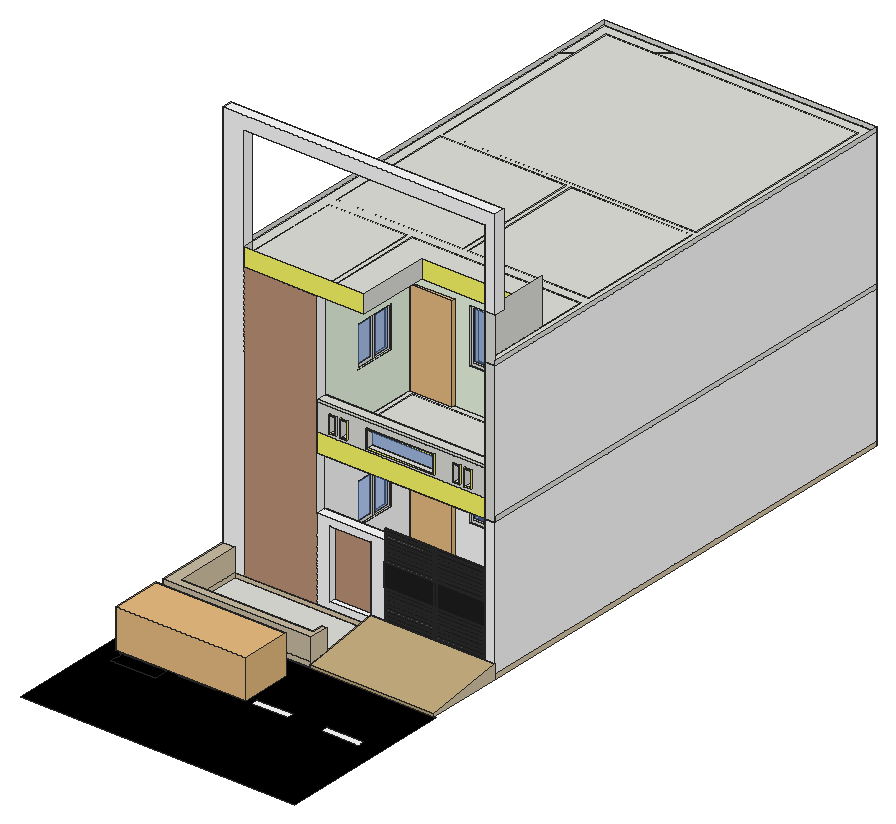
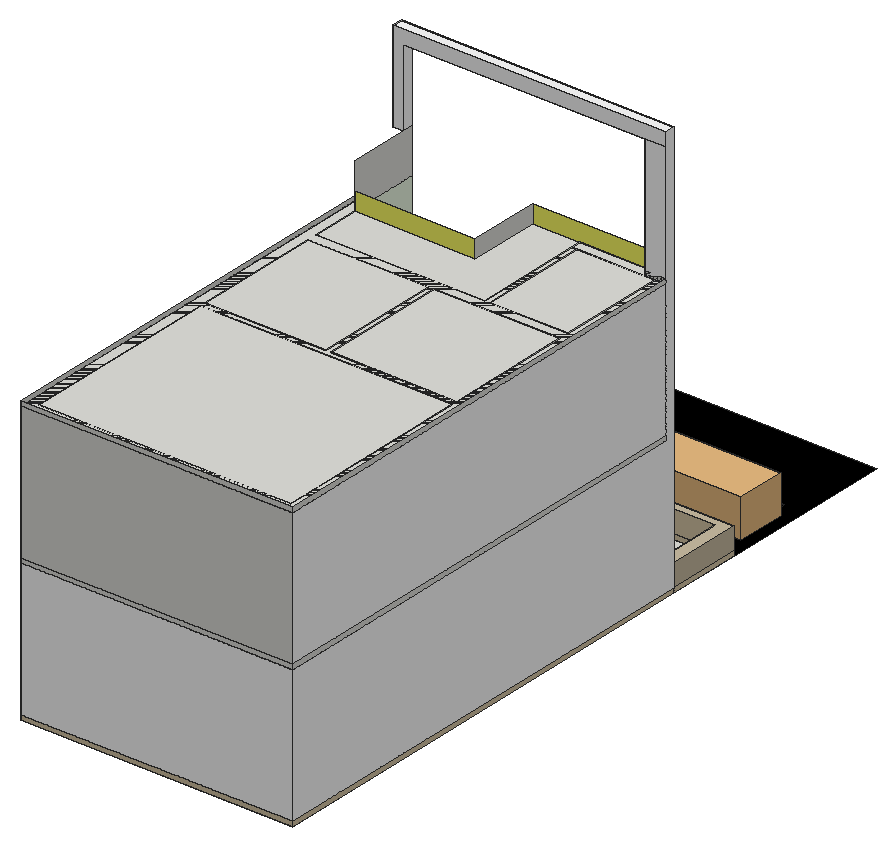
# SketchUp Ruby script. Lengths in inches.
U = 1.inch
M = Sketchup.active_model
def pt(a) = Geom::Point3d.new(a.map { |v| v * U })
def face(e, loops, mat)
  f = e.add_face(loops[0].map { |a| pt(a) })
  loops[1..].each { |l| e.add_face(l.map { |a| pt(a) }).erase! }
  f.material = f.back_material = mat if mat
  f
end
# faces: each face lists its corners as indices into pts; further lists are holes
def faces(e, pts, list, mat = nil) = list.each { |f| face(e, (f[0].is_a?(Array) ? f : [f]).map { |l| l.map { |i| pts[i] } }, mat) }
# xy, xz, yz: faces in a plane at the given z, y or x. An outline is a flat list of corners, or four numbers for a rectangle; further outlines are holes
def ring(l) = l.size == 4 ? [[l[0], l[1]], [l[2], l[1]], [l[2], l[3]], [l[0], l[3]]] : l.each_slice(2).to_a
def flat(e, list, mat, &to3) = list.each { |f| face(e, (f[0].is_a?(Array) ? f : [f]).map { |l| ring(l).map { |u, v| to3.(u, v) } }, mat) }
def xy(e, z, list, mat = nil) = flat(e, list, mat) { |x, y| [x, y, z] }
def xz(e, y, list, mat = nil) = flat(e, list, mat) { |x, z| [x, y, z] }
def yz(e, x, list, mat = nil) = flat(e, list, mat) { |y, z| [x, y, z] }
def lines(e, pts, list) = list.each { |a, b| e.add_line(pt(pts[a]), pt(pts[b])) }
# prism: a flat outline (further loops are holes) pulled along v
def prism(e, loops, v, mat = nil)
  f = face(e, loops, mat); d = Geom::Vector3d.new(v.map { |x| x * U })
  f.pushpull(f.normal.samedirection?(d) ? d.length : -d.length)
end
def box(e, o, s, mat = nil) = prism(e, [[o, [o[0] + s[0], o[1], o[2]], [o[0] + s[0], o[1] + s[1], o[2]], [o[0], o[1] + s[1], o[2]]]], [0, 0, s[2]], mat)
def at(x, y, z, deg = 0) = Geom::Transformation.translation(pt([x, y, z])) * Geom::Transformation.rotation(ORIGIN, Z_AXIS, deg.degrees)
def axes(o, x, y, z) = Geom::Transformation.new([*x, 0, *y, 0, *z, 0, *pt(o).to_a, 1])
def part(name) = M.definitions.add(name)
# library, detail: a bought-in or finely detailed component or shape, given as its bounding box
def library(name, o, s) = part(name).tap { |d| box(d.entities, o, s) }
def detail(e, o, s) = box(e.add_group.entities, o, s)
def put(e, d, t, mat = nil) = e.add_instance(d, t).tap { |i| i.material = mat if mat }
def group(e, t, mat = nil) = e.add_group.tap { |g| g.transformation = t; g.material = mat if mat }.entities
root = M.entities
M.materials.add("Color_008").color = [30, 30, 30]
M.materials.add("[0055_LightGoldenrodYellow]").color = [250, 250, 210]
M.materials.add("[0131_Silver]").color = [192, 192, 192]
M.materials.add("[0134_DimGray]").color = [105, 105, 105]
M.materials.add("[Color A01]").color = [191, 147, 119]
M.materials.add("[Color C01]").color = [191, 147, 119]
M.materials.add("[Color E03]").color = [255, 255, 104]
M.materials.add("[Color M00]").color = [255, 255, 255]
M.materials.add("[Color M09]").color = [0, 0, 0]
M.materials.add("[Concrete Tile]").color = [203, 190, 164]
M.materials.add("[Field Square Tile]").color = [217, 201, 169]
M.materials.add("[Roofing Slate Tan]").color = [200, 175, 128]
M.materials.add("[Tile Limestone Large]").color = [238, 251, 230]
M.materials.add("[Translucent Glass Blue]").color = [100, 149, 237]
M.materials["[Translucent Glass Blue]"].alpha = 0.5
c1 = library("Passenger car",[0,0,0],[114.57,43.85,34.01])
c2 = library("Untitled",[-28.23,109.14,0],[52,7.35,84])
c3 = part("Gate slat")
box(c3.entities,[0,0,-2.03],[1.97,0.97,40.94])
c4 = part("Gate frame member")
box(c4.entities,[0,0,0],[1.9,0.97,93.54])
c5 = part("Gate slat \#1")
box(c5.entities,[2.95,0,-2.03],[0.99,0.97,40.94])
c6 = part("Slatted gate")
p = [[42.85,0.97,43.31],[42.85,0.97,44.29]]
lines(c6.entities,p,[[0,1]])
put(c6.entities,c3,axes([3.9375,0,86.61],[0,0,-1],[0,1,0],[1,0,0]),"Color_008")
put(c6.entities,c4,axes([87.6,0,0],[1,0,0],[0,1,0],[0,0,0.92593]),"Color_008")
put(c6.entities,c3,axes([48.6875,0,86.61],[0,0,-1],[0,1,0],[1,0,0]),"Color_008")
put(c6.entities,c4,axes([0,0,0],[1,0,0],[0,1,0],[0,0,0.92593]),"Color_008")
put(c6.entities,c4,axes([42.85,0,0],[1,0,0],[0,1,0],[0,0,0.92593]),"Color_008")
put(c6.entities,c4,axes([44.75,0,0],[1,0,0],[0,1,0],[0,0,0.92593]),"Color_008")
put(c6.entities,c5,axes([3.9375,0,87.11],[0,0,-1],[0,1,0],[1,0,0]),"[0134_DimGray]")
put(c6.entities,c5,axes([48.6875,0,87.11],[0,0,-1],[0,1,0],[1,0,0]),"[0134_DimGray]")
put(c6.entities,c3,axes([48.6875,0,82.68],[0,0,-1],[0,1,0],[1,0,0]),"Color_008")
put(c6.entities,c5,axes([48.6875,0,83.17],[0,0,-1],[0,1,0],[1,0,0]),"[0134_DimGray]")
put(c6.entities,c5,axes([3.9375,0,83.17],[0,0,-1],[0,1,0],[1,0,0]),"[0134_DimGray]")
put(c6.entities,c3,axes([3.9375,0,82.68],[0,0,-1],[0,1,0],[1,0,0]),"Color_008")
put(c6.entities,c5,axes([48.6875,0,75.3],[0,0,-1],[0,1,0],[1,0,0]),"[0134_DimGray]")
put(c6.entities,c3,axes([48.6875,0,78.74],[0,0,-1],[0,1,0],[1,0,0]),"Color_008")
put(c6.entities,c3,axes([48.6875,0,74.8],[0,0,-1],[0,1,0],[1,0,0]),"Color_008")
put(c6.entities,c5,axes([48.6875,0,79.23],[0,0,-1],[0,1,0],[1,0,0]),"[0134_DimGray]")
put(c6.entities,c5,axes([3.9375,0,75.3],[0,0,-1],[0,1,0],[1,0,0]),"[0134_DimGray]")
put(c6.entities,c3,axes([3.9375,0,78.74],[0,0,-1],[0,1,0],[1,0,0]),"Color_008")
put(c6.entities,c5,axes([3.9375,0,79.23],[0,0,-1],[0,1,0],[1,0,0]),"[0134_DimGray]")
put(c6.entities,c3,axes([3.9375,0,74.8],[0,0,-1],[0,1,0],[1,0,0]),"Color_008")
put(c6.entities,c5,axes([48.6875,0,67.42],[0,0,-1],[0,1,0],[1,0,0]),"[0134_DimGray]")
put(c6.entities,c5,axes([3.9375,0,63.48],[0,0,-1],[0,1,0],[1,0,0]),"[0134_DimGray]")
put(c6.entities,c5,axes([48.6875,0,71.36],[0,0,-1],[0,1,0],[1,0,0]),"[0134_DimGray]")
put(c6.entities,c5,axes([3.9375,0,67.42],[0,0,-1],[0,1,0],[1,0,0]),"[0134_DimGray]")
put(c6.entities,c3,axes([3.9375,0,70.87],[0,0,-1],[0,1,0],[1,0,0]),"Color_008")
put(c6.entities,c3,axes([48.6875,0,70.87],[0,0,-1],[0,1,0],[1,0,0]),"Color_008")
put(c6.entities,c3,axes([48.6875,0,66.93],[0,0,-1],[0,1,0],[1,0,0]),"Color_008")
put(c6.entities,c3,axes([48.6875,0,59.06],[0,0,-1],[0,1,0],[1,0,0]),"Color_008")
put(c6.entities,c3,axes([3.9375,0,55.12],[0,0,-1],[0,1,0],[1,0,0]),"Color_008")
put(c6.entities,c3,axes([3.9375,0,62.99],[0,0,-1],[0,1,0],[1,0,0]),"Color_008")
put(c6.entities,c5,axes([3.9375,0,59.55],[0,0,-1],[0,1,0],[1,0,0]),"[0134_DimGray]")
put(c6.entities,c3,axes([3.9375,0,66.93],[0,0,-1],[0,1,0],[1,0,0]),"Color_008")
put(c6.entities,c3,axes([48.6875,0,62.99],[0,0,-1],[0,1,0],[1,0,0]),"Color_008")
put(c6.entities,c5,axes([48.6875,0,59.55],[0,0,-1],[0,1,0],[1,0,0]),"[0134_DimGray]")
put(c6.entities,c5,axes([48.6875,0,63.48],[0,0,-1],[0,1,0],[1,0,0]),"[0134_DimGray]")
put(c6.entities,c3,axes([3.9375,0,59.06],[0,0,-1],[0,1,0],[1,0,0]),"Color_008")
put(c6.entities,c5,axes([3.9375,0,71.36],[0,0,-1],[0,1,0],[1,0,0]),"[0134_DimGray]")
put(c6.entities,c5,axes([3.9375,0,33.96],[0,0,-1],[0,1,0],[1,0,0]),"[0134_DimGray]")
put(c6.entities,c5,axes([48.6875,0,33.96],[0,0,-1],[0,1,0],[1,0,0]),"[0134_DimGray]")
put(c6.entities,c3,axes([3.9375,0,29.53],[0,0,-1],[0,1,0],[1,0,0]),"Color_008")
put(c6.entities,c5,axes([3.9375,0,26.08],[0,0,-1],[0,1,0],[1,0,0]),"[0134_DimGray]")
put(c6.entities,c3,axes([3.9375,0,33.46],[0,0,-1],[0,1,0],[1,0,0]),"Color_008")
put(c6.entities,c3,axes([48.6875,0,29.53],[0,0,-1],[0,1,0],[1,0,0]),"Color_008")
put(c6.entities,c5,axes([48.6875,0,30.02],[0,0,-1],[0,1,0],[1,0,0]),"[0134_DimGray]")
put(c6.entities,c3,axes([3.9375,0,25.59],[0,0,-1],[0,1,0],[1,0,0]),"Color_008")
put(c6.entities,c3,axes([48.6875,0,25.59],[0,0,-1],[0,1,0],[1,0,0]),"Color_008")
put(c6.entities,c3,axes([48.6875,0,33.46],[0,0,-1],[0,1,0],[1,0,0]),"Color_008")
put(c6.entities,c3,axes([3.9375,0,49.7],[0,0,-1],[0,1,0],[1,0,0]),"Color_008")
put(c6.entities,c5,axes([48.6875,0,26.08],[0,0,-1],[0,1,0],[1,0,0]),"[0134_DimGray]")
put(c6.entities,c5,axes([3.9375,0,30.02],[0,0,-1],[0,1,0],[1,0,0]),"[0134_DimGray]")
put(c6.entities,c3,axes([3.9375,0,5.91],[0,0,-1],[0,1,0],[1,0,0]),"Color_008")
put(c6.entities,c3,axes([48.6875,0,13.78],[0,0,-1],[0,1,0],[1,0,0]),"Color_008")
put(c6.entities,c5,axes([48.6875,0,10.33],[0,0,-1],[0,1,0],[1,0,0]),"[0134_DimGray]")
put(c6.entities,c5,axes([3.9375,0,6.4],[0,0,-1],[0,1,0],[1,0,0]),"[0134_DimGray]")
put(c6.entities,c3,axes([3.9375,0,13.78],[0,0,-1],[0,1,0],[1,0,0]),"Color_008")
put(c6.entities,c3,axes([48.6875,0,21.65],[0,0,-1],[0,1,0],[1,0,0]),"Color_008")
put(c6.entities,c3,axes([48.6875,0,5.91],[0,0,-1],[0,1,0],[1,0,0]),"Color_008")
put(c6.entities,c5,axes([48.6875,0,22.15],[0,0,-1],[0,1,0],[1,0,0]),"[0134_DimGray]")
put(c6.entities,c3,axes([48.6875,0,1.97],[0,0,-1],[0,1,0],[1,0,0]),"Color_008")
put(c6.entities,c3,axes([48.6875,0,9.84],[0,0,-1],[0,1,0],[1,0,0]),"Color_008")
put(c6.entities,c5,axes([48.6875,0,6.4],[0,0,-1],[0,1,0],[1,0,0]),"[0134_DimGray]")
put(c6.entities,c3,axes([3.9375,0,9.84],[0,0,-1],[0,1,0],[1,0,0]),"Color_008")
put(c6.entities,c5,axes([3.9375,0,10.33],[0,0,-1],[0,1,0],[1,0,0]),"[0134_DimGray]")
put(c6.entities,c5,axes([3.9375,0,22.15],[0,0,-1],[0,1,0],[1,0,0]),"[0134_DimGray]")
put(c6.entities,c3,axes([3.9375,0,1.97],[0,0,-1],[0,1,0],[1,0,0]),"Color_008")
put(c6.entities,c5,axes([3.9375,0,18.21],[0,0,-1],[0,1,0],[1,0,0]),"[0134_DimGray]")
put(c6.entities,c5,axes([3.9375,0,14.27],[0,0,-1],[0,1,0],[1,0,0]),"[0134_DimGray]")
put(c6.entities,c3,axes([3.9375,0,21.65],[0,0,-1],[0,1,0],[1,0,0]),"Color_008")
put(c6.entities,c5,axes([48.6875,0,18.21],[0,0,-1],[0,1,0],[1,0,0]),"[0134_DimGray]")
put(c6.entities,c3,axes([3.9375,0,17.72],[0,0,-1],[0,1,0],[1,0,0]),"Color_008")
put(c6.entities,c3,axes([48.6875,0,17.72],[0,0,-1],[0,1,0],[1,0,0]),"Color_008")
put(c6.entities,c5,axes([48.6875,0,14.27],[0,0,-1],[0,1,0],[1,0,0]),"[0134_DimGray]")
put(c6.entities,c3,axes([3.9375,0,44.29],[0,0,-1],[0,1,0],[1,0,0]),"Color_008")
put(c6.entities,c3,axes([3.9375,0,38.88],[0,0,-1],[0,1,0],[1,0,0]),"Color_008")
put(c6.entities,c3,axes([48.6875,0,49.7],[0,0,-1],[0,1,0],[1,0,0]),"Color_008")
put(c6.entities,c3,axes([48.6875,0,44.29],[0,0,-1],[0,1,0],[1,0,0]),"Color_008")
put(c6.entities,c3,axes([48.6875,0,38.88],[0,0,-1],[0,1,0],[1,0,0]),"Color_008")
put(c6.entities,c3,axes([48.6875,0,55.12],[0,0,-1],[0,1,0],[1,0,0]),"Color_008")
c7 = part("Glass panel \#1")
box(c7.entities,[0,0,-1.97],[52.81,0.39,23.62])
c8 = part("Glass panel")
box(c8.entities,[0,0,-9.84],[39.64,0.39,36.58])
c9 = part("Janela aluminio")
xy(c9.entities,0,[[0,0,47.24,1.57],[23.62,1.57,47.24,2.76],[0,2.76,25.98,3.9375],[0,3.9375,47.24,5.91]])
xy(c9.entities,43.31,[[0,0,47.24,1.57],[23.62,1.57,47.24,2.76],[0,2.76,0,5.91,47.24,5.91,47.24,3.9375,25.98,3.9375,25.98,2.76],[25.98,2.76,47.24,3.9375]])
xz(c9.entities,1.57,[[0,0,23.62,0,23.62,41.34,21.26,41.34,21.26,1.97,1.97,1.97,1.97,41.34,23.62,41.34,23.62,43.31,0,43.31],[[23.62,0,47.24,43.31],[25.7,1.97,45.28,41.34]]])
xz(c9.entities,2.76,[[[0,0,23.62,43.31],[2.36,2.36,21.26,40.94]],[23.62,0,25.98,43.31]])
xz(c9.entities,2.76,[[2.36,2.36,21.26,40.94]],"[Translucent Glass Blue]")
xz(c9.entities,3.9375,[[25.98,0,25.98,2.36,44.88,2.36,44.88,40.94,25.98,40.94,25.98,43.31,47.24,43.31,47.24,0]])
xz(c9.entities,3.9375,[[25.98,2.36,44.88,40.94]],"[Translucent Glass Blue]")
yz(c9.entities,0,[[0,0,1.57,43.31],[2.76,0,5.91,43.31]])
yz(c9.entities,23.62,[[1.57,0,2.76,43.31]])
yz(c9.entities,25.98,[[2.76,0,3.9375,43.31]])
yz(c9.entities,47.24,[[0,0,1.57,43.31],[1.57,0,2.76,43.31],[3.9375,0,5.91,43.31]])
xy(root,19.1,[[0,156,130.5,223.5]])
xy(root,19.1,[[66.31,91.44,99.35,98.41],[14.46,91.5,47.5,98.47],[129.67,91.8125,162.71,98.78],[191.22,91.96,224.26,98.93]],"[Color M00]")
xy(root,19.1,[[[0,0,242,156],[16.76,78.5,16.76,91.5,14.46,91.5,14.46,98.47,47.5,98.47,47.5,91.5,56.26,91.5,56.26,78.5],[66.31,91.44,99.35,98.41],[129.67,91.8125,162.71,98.78],[191.22,91.96,224.26,98.93]],[16.76,78.5,56.26,91.5]],"[Color M09]")
xy(root,267.1,[[18,223.5,18,232.5,0,232.5,0,643.5,240,643.5,240,223.5,231,223.5,231,286.5,124.5,286.5,124.5,223.5]])
xz(root,223.5,[[231,267.1,240,307.1]])
xz(root,223.5,[[18,267.1,124.5,283.1]],"[Color E03]")
xz(root,232.5,[[0,267.1,18,271.1]])
xz(root,286.5,[[124.5,267.1,231,283.1]],"[Color E03]")
xz(root,643.5,[[0,267.1,240,271.1]])
yz(root,0,[[232.5,267.1,643.5,271.1]])
yz(root,18,[[223.5,267.1,232.5,283.1]])
yz(root,124.5,[[223.5,267.1,286.5,283.1]])
yz(root,231,[[223.5,267.1,286.5,307.1]])
yz(root,240,[[223.5,267.1,643.5,271.1]])
p = [[231,223.5,143.1],[231,223.5,147.1],[240,223.5,147.1],[240,223.5,143.1]]
lines(root,p,[[0,1],[2,3],[3,0]])
g1 = group(root,at(0,223.5,23.1),"[Field Square Tile]")
xy(g1,-4,[[130.5,-67.5,240,0],[0,-66,0,0,10.75,0,10.75,-59,130.5,-59,130.5,-66],[0,0,240,420]])
xy(g1,0,[[126.5,-59,130.5,-49]])
xy(g1,20,[[0,-66,130.5,-66,130.5,-49,126.5,-49,126.5,-59,10.75,-59,10.75,0,0,0]],"[Concrete Tile]")
xz(g1,-66,[[0,-4,130.5,0],[0,0,130.5,20]],"[Concrete Tile]")
xz(g1,-59,[[10.75,-4,130.5,0],[10.75,0,126.5,20]])
xz(g1,-49,[[126.5,0,130.5,20]])
xz(g1,0,[[0,-4,10.75,0],[10.75,-4,130.5,0],[130.5,-4,240,6],[0,0,10.75,20]])
xz(g1,420,[[0,-4,240,0]])
yz(g1,0,[[-66,-4,0,0],[0,-4,420,0]])
yz(g1,0,[[-66,0,0,20]],"[Concrete Tile]")
yz(g1,10.75,[[-59,-4,0,0],[-59,0,0,20]])
yz(g1,126.5,[[-59,0,-49,20]])
yz(g1,130.5,[[-67.5,-4,-67.87,-1.53,-66,-1.25,-66,-4],[-66,-4,-59,-4,-59,-0.21,-66,-1.25],[-66,-1.25,-59,-0.21,-59,0,-57.56,0,-49,1.27,-49,20,-66,20],[-57.56,0,-49,1.27,-49,0]])
yz(g1,130.5,[[-59,-4,-59,-0.21,-57.56,0,-49,0,-49,1.27,-0.37,8.47,0,6,0,-4]],"[Roofing Slate Tan]")
yz(g1,240,[[-67.5,-4,0,-4,0,6,-0.37,8.47,-67.87,-1.53],[0,-4,420,0]])
p = [[130.5,-67.5,-4],[240,-67.5,-4],[240,-67.87,-1.53],[130.5,-67.87,-1.53],[130.5,-0.37,8.47],[130.5,-49,1.27],
  [130.5,-57.56,0],[130.5,-59,-0.21],[130.5,-66,-1.25],[240,-0.37,8.47],[240,0,6],[130.5,0,6]]
faces(g1,p,[[0,1,2,3],[4,5,6,7,8,3,2,9]],"[Roofing Slate Tan]")
faces(g1,p,[[10,11,4,9]])
put(root,c1,at(124.73,136.77,19.1,-180))
put(root,c2,axes([211.8,216.7,23.1],[0.80769,0,0],[0,1,0],[0,0,1]))
put(root,c2,axes([102.86,216.7,23.1],[0.72115,0,0],[0,1,0],[0,0,1]))
g2 = group(root,at(0,223.5,23.1))
xy(g2,0,[[[0,0,0,420,240,420,240,0,231,0,231,228,124.5,228,124.5,114,172.5,114,172.5,105,120,105,120,228,9,228,9,114,82.5,114,82.5,9,142.5,9,142.5,0],[9,232.5,231,411],[9,9,78,105]],[172.5,105,189,114]],"[Color M00]")
xy(g2,6,[[94.5,0,130.5,5]],"[Color M00]")
xy(g2,36,[[133.5,105,172.5,114]],"[Color M00]")
xy(g2,42,[[78,45,82.5,81]],"[Color M00]")
xy(g2,66,[[94.5,0,130.5,5]],"[Color M00]")
xy(g2,72,[[82.5,0,142.5,9]],"[Color M00]")
xy(g2,78,[[78,45,82.5,81]],"[Color M00]")
xy(g2,84,[[82.5,105,120,114],[133.5,105,172.5,114],[189,105,231,114]],"[Color M00]")
xy(g2,120,[[[231,0,240,0,240,420,0,420,0,9,9,9,9,105,78,105,78,9,82.5,9,82.5,105,231,105,231,114,124.5,114,124.5,228,231,228],[9,232.5,231,411],[9,114,120,228]],[9,9,78,105]],"[Color M00]")
xy(g2,244,[[18,0,82.5,9]],"[Color M00]")
xy(g2,284,[[231,0,240,9]],"[Color M00]")
xy(g2,352,[[18,0,231,9]],"[Color M00]")
xy(g2,364,[[0,0,240,9]],"[Color M00]")
xz(g2,0,[[18,0,82.5,244]],"[Color C01]")
xz(g2,0,[[0,0,18,0,18,352,231,352,231,284,240,284,240,364,0,364],[[82.5,0,142.5,72],[94.5,6,130.5,66]],[231,0,240,120]],"[Color M00]")
xz(g2,5,[[94.5,6,130.5,66]],"[Color A01]")
xz(g2,9,[[9,0,78,120],[82.5,0,142.5,72],[0,120,0,352,18,352,18,244,78,244,78,120],[78,120,82.5,244],[231,284,231,352,0,352,0,364,240,364,240,284]],"[Color M00]")
xz(g2,45,[[78,42,82.5,78]],"[Color M00]")
xz(g2,81,[[78,42,82.5,78]],"[Color M00]")
xz(g2,105,[[9,0,78,120],[120,0,172.5,0,172.5,36,133.5,36,133.5,84,172.5,84,172.5,0,189,0,189,84,231,84,231,120,82.5,120,82.5,84,120,84]],"[Color M00]")
xz(g2,114,[[9,0,9,120,120,120,120,84,82.5,84,82.5,0],[[124.5,0,124.5,120,231,120,231,84,189,84,189,0],[133.5,36,172.5,84]]],"[Color M00]")
xz(g2,228,[[9,0,120,120],[124.5,0,231,120]],"[Color M00]")
xz(g2,232.5,[[9,0,231,120]],"[Color M00]")
xz(g2,411,[[9,0,231,120]],"[Color M00]")
xz(g2,420,[[0,0,240,120]],"[Color M00]")
yz(g2,0,[[0,0,0,364,9,364,9,120,420,120,420,0]],"[Color M00]")
yz(g2,9,[[9,0,105,120],[114,0,228,120],[232.5,0,411,120]],"[Color M00]")
yz(g2,18,[[0,244,9,352]],"[Color M00]")
yz(g2,78,[[9,0,9,120,81,120,81,78,45,78,45,42,81,42,81,0],[81,0,105,120]],"[Color M00]")
yz(g2,82.5,[[[9,0,114,0,114,84,105,84,105,120,9,120],[45,42,81,78]],[0,72,9,244]],"[Color M00]")
yz(g2,94.5,[[0,6,5,66]],"[Color M00]")
yz(g2,120,[[105,0,105,84,114,84,114,120,228,120,228,0]],"[Color M00]")
yz(g2,124.5,[[114,0,228,120]],"[Color M00]")
yz(g2,130.5,[[0,6,5,66]],"[Color M00]")
yz(g2,133.5,[[105,36,114,84]],"[Color M00]")
yz(g2,142.5,[[0,0,9,72]],"[Color M00]")
yz(g2,172.5,[[105,36,114,84]],"[Color M00]")
yz(g2,189,[[105,0,114,84]],"[Color M00]")
yz(g2,231,[[0,0,0,120,105,120,105,84,114,84,114,120,228,120,228,0],[232.5,0,411,120],[0,284,9,352]],"[Color M00]")
yz(g2,240,[[0,0,420,120],[0,284,9,364]],"[Color M00]")
g3 = group(root,at(142.65,222.74,31.58))
put(g3,c6,axes([0,0.39,0],[0.9871,0,0],[0,1,0],[0,0,0.83731]),"[0055_LightGoldenrodYellow]")
put(g3,c7,axes([0,0,28.02],[0.83651,0,0],[0,1,0],[0,0,0.83731]),"Color_008")
put(g3,c8,axes([44.17,1.36,52.8],[1.0671,0,0],[0,1,0],[0,0,0.67588]),"[0131_Silver]")
put(g3,c8,axes([1.88,1.36,8.3],[1.0671,0,0],[0,1,0],[0,0,0.67588]),"[0131_Silver]")
put(g3,c8,axes([1.88,1.36,52.8],[1.0671,0,0],[0,1,0],[0,0,0.67588]),"[0131_Silver]")
put(g3,c7,axes([44.17,0,28.02],[0.83651,0,0],[0,1,0],[0,0,0.83731]),"Color_008")
put(g3,c8,axes([44.17,1.36,8.3],[1.0671,0,0],[0,1,0],[0,0,0.67588]),"[0131_Silver]")
put(root,c9,axes([133.5,328.5,59.1],[0.8255,0,0],[0,1,0],[0,0,1.10836]))
put(root,c9,axes([79.41,268.5,65.1],[0,0.75438,0],[0.6325,0,0],[0,0,0.83127]))
g4 = group(root,at(0,223.5,147.1))
xy(g4,0,[[172.5,105,189,114]])
xy(g4,36,[[133.5,105,172.5,114]])
xy(g4,42,[[78,45,82.5,81]])
xy(g4,78,[[78,45,82.5,81]])
xy(g4,84,[[82.5,105,120,114],[133.5,105,172.5,114],[189,105,231,114]])
xy(g4,120,[[[231,0,240,0,240,420,0,420,0,9,9,9,9,105,78,105,78,9,82.5,9,82.5,105,231,105,231,114,124.5,114,124.5,228,231,228],[9,232.5,231,411],[9,114,120,228]]])
xz(g4,0,[[231,-4,240,120]])
xz(g4,9,[[0,0,9,120],[9,0,78,120],[78,0,82.5,120]])
xz(g4,45,[[78,42,82.5,78]])
xz(g4,81,[[78,42,82.5,78]])
xz(g4,105,[[9,0,78,120]])
xz(g4,105,[[120,0,172.5,0,172.5,36,133.5,36,133.5,84,172.5,84,172.5,0,189,0,189,84,231,84,231,120,82.5,120,82.5,84,120,84]],"[Tile Limestone Large]")
xz(g4,114,[[9,0,9,120,120,120,120,84,82.5,84,82.5,0],[[124.5,0,124.5,120,231,120,231,84,189,84,189,0],[133.5,36,172.5,84]]])
xz(g4,228,[[9,0,120,120],[124.5,0,231,120]])
xz(g4,232.5,[[9,0,231,120]])
xz(g4,411,[[9,0,231,120]])
xz(g4,420,[[0,0,240,120]])
yz(g4,0,[[9,0,420,120]],"[Color M00]")
yz(g4,9,[[9,0,105,120],[114,0,228,120],[232.5,0,411,120]])
yz(g4,78,[[9,0,9,120,81,120,81,78,45,78,45,42,81,42,81,0],[81,0,105,120]])
yz(g4,82.5,[[[9,0,114,0,114,84,105,84,105,120,9,120],[45,42,81,78]]],"[Tile Limestone Large]")
yz(g4,120,[[105,0,105,84,114,84,114,120,228,120,228,0]])
yz(g4,124.5,[[114,0,228,120]])
yz(g4,133.5,[[105,36,114,84]])
yz(g4,172.5,[[105,36,114,84]])
yz(g4,189,[[105,0,114,84]])
yz(g4,231,[[232.5,0,411,120]])
yz(g4,231,[[0,0,0,120,105,120,105,84,114,84,114,120,228,120,228,0]],"[Tile Limestone Large]")
yz(g4,240,[[0,0,420,120]],"[Color M00]")
g5 = group(root,at(0,223.5,147.1))
xy(g5,-4,[[82.5,0,82.5,9,0,9,0,420,240,420,240,0]])
xy(g5,12,[[82.5,0,231,9]])
xy(g5,15,[[126.98,-1,186.5,0]])
xy(g5,15.5,[[94,-1,100,0],[203.5,-1,209.5,0],[213.5,-1,219.5,0]])
xy(g5,15.52,[[104.02,-1,109.98,0]])
xy(g5,16,[[94.5,-1,99.5,9],[104.5,-1,109.5,9],[127.98,-1,185.5,4],[204,-1,209,9],[214,-1,219,9]])
xy(g5,30,[[94.5,-1,99.5,9],[104.5,-1,109.5,9],[127.98,-1,185.5,4],[204,-1,209,9],[214,-1,219,9]])
xy(g5,30.48,[[104.02,-1,109.98,0]],"[Color E03]")
xy(g5,30.5,[[94,-1,100,0],[203.5,-1,209.5,0],[213.5,-1,219.5,0]],"[Color E03]")
xy(g5,31,[[126.98,-1,186.5,0]],"[Color E03]")
xy(g5,36,[[82.5,0,231,9]])
xy(g5,38,[[82.5,0,231,9]])
xz(g5,-1,[[[126.98,15,186.5,31],[127.98,16,185.5,30]],[[94,15.5,100,30.5],[94.5,16,99.5,30]],[[203.5,15.5,209.5,30.5],[204,16,209,30]],[[213.5,15.5,219.5,30.5],[214,16,219,30]],[[104.02,15.52,109.98,30.48],[104.5,16,109.5,30]]],"[Color E03]")
xz(g5,0,[[[82.5,12,231,36],[126.98,15,186.5,31],[94,15.5,100,30.5],[203.5,15.5,209.5,30.5],[213.5,15.5,219.5,30.5],[104.02,15.52,109.98,30.48]],[82.5,36,231,38]])
xz(g5,0,[[82.5,-4,231,12]],"[Color E03]")
xz(g5,4,[[127.98,16,185.5,30]],"[Translucent Glass Blue]")
xz(g5,9,[[0,-4,82.5,0],[82.5,0,231,12],[[82.5,12,231,36],[94.5,16,99.5,30],[104.5,16,109.5,30],[204,16,209,30],[214,16,219,30]],[82.5,36,231,38]])
xz(g5,420,[[0,-4,240,0]])
yz(g5,0,[[9,-4,420,0]])
yz(g5,82.5,[[0,-4,9,12],[0,12,9,36],[0,36,9,38]])
yz(g5,94,[[-1,15.5,0,30.5]],"[Color E03]")
yz(g5,94.5,[[-1,16,9,30]])
yz(g5,99.5,[[-1,16,9,30]])
yz(g5,100,[[-1,15.5,0,30.5]])
yz(g5,104.02,[[-1,15.52,0,30.48]],"[Color E03]")
yz(g5,104.5,[[-1,16,9,30]])
yz(g5,109.5,[[-1,16,9,30]])
yz(g5,109.98,[[-1,15.52,0,30.48]],"[Color E03]")
yz(g5,126.98,[[-1,15,0,31]],"[Color E03]")
yz(g5,127.98,[[-1,16,4,30]])
yz(g5,185.5,[[-1,16,4,30]])
yz(g5,186.5,[[-1,15,0,31]],"[Color E03]")
yz(g5,203.5,[[-1,15.5,0,30.5]],"[Color E03]")
yz(g5,204,[[-1,16,9,30]])
yz(g5,209,[[-1,16,9,30]])
yz(g5,209.5,[[-1,15.5,0,30.5]],"[Color E03]")
yz(g5,213.5,[[-1,15.5,0,30.5]],"[Color E03]")
yz(g5,214,[[-1,16,9,30]])
yz(g5,219,[[-1,16,9,30]])
yz(g5,219.5,[[-1,15.5,0,30.5]],"[Color E03]")
yz(g5,231,[[0,0,9,12],[0,12,9,36],[0,36,9,38]])
yz(g5,240,[[0,-4,420,0]])
put(root,c2,axes([102.86,216.7,147.1],[0.72115,0,0],[0,1,0],[0,0,1]))
put(root,c2,axes([211.8,216.7,147.1],[0.80769,0,0],[0,1,0],[0,0,1]))
put(root,c9,axes([133.5,328.5,183.1],[0.8255,0,0],[0,1,0],[0,0,1.10836]))
put(root,c9,axes([79.41,268.5,189.1],[0,0.75438,0],[0.6325,0,0],[0,0,0.83127]))
